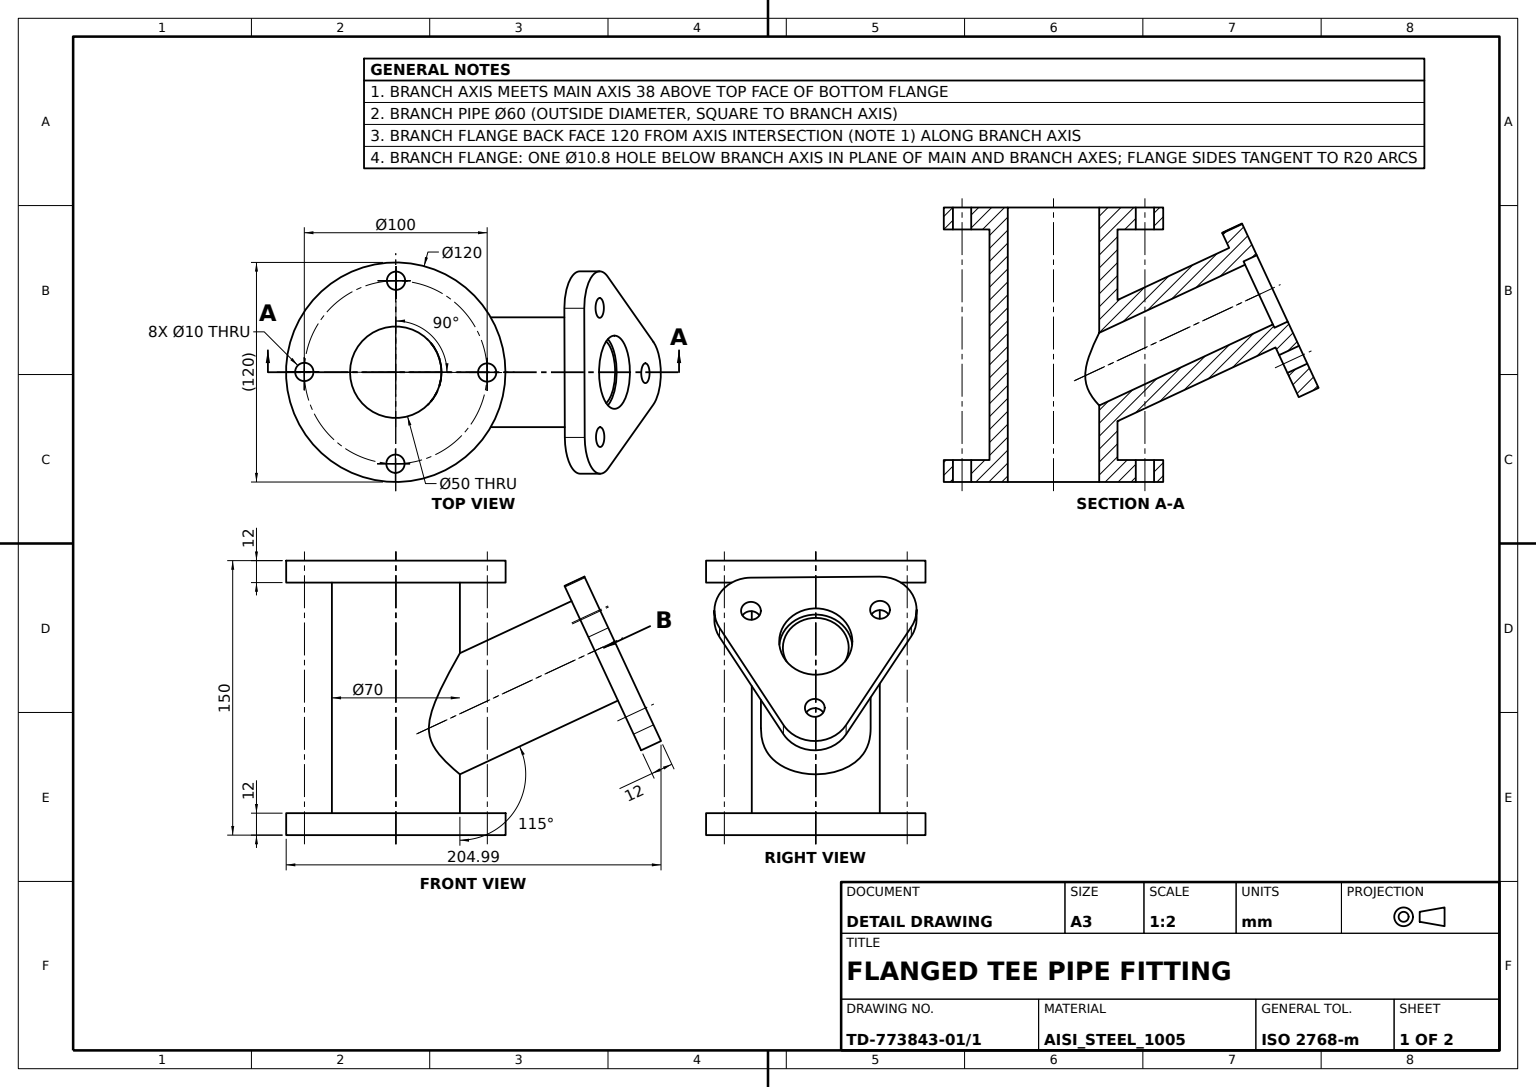
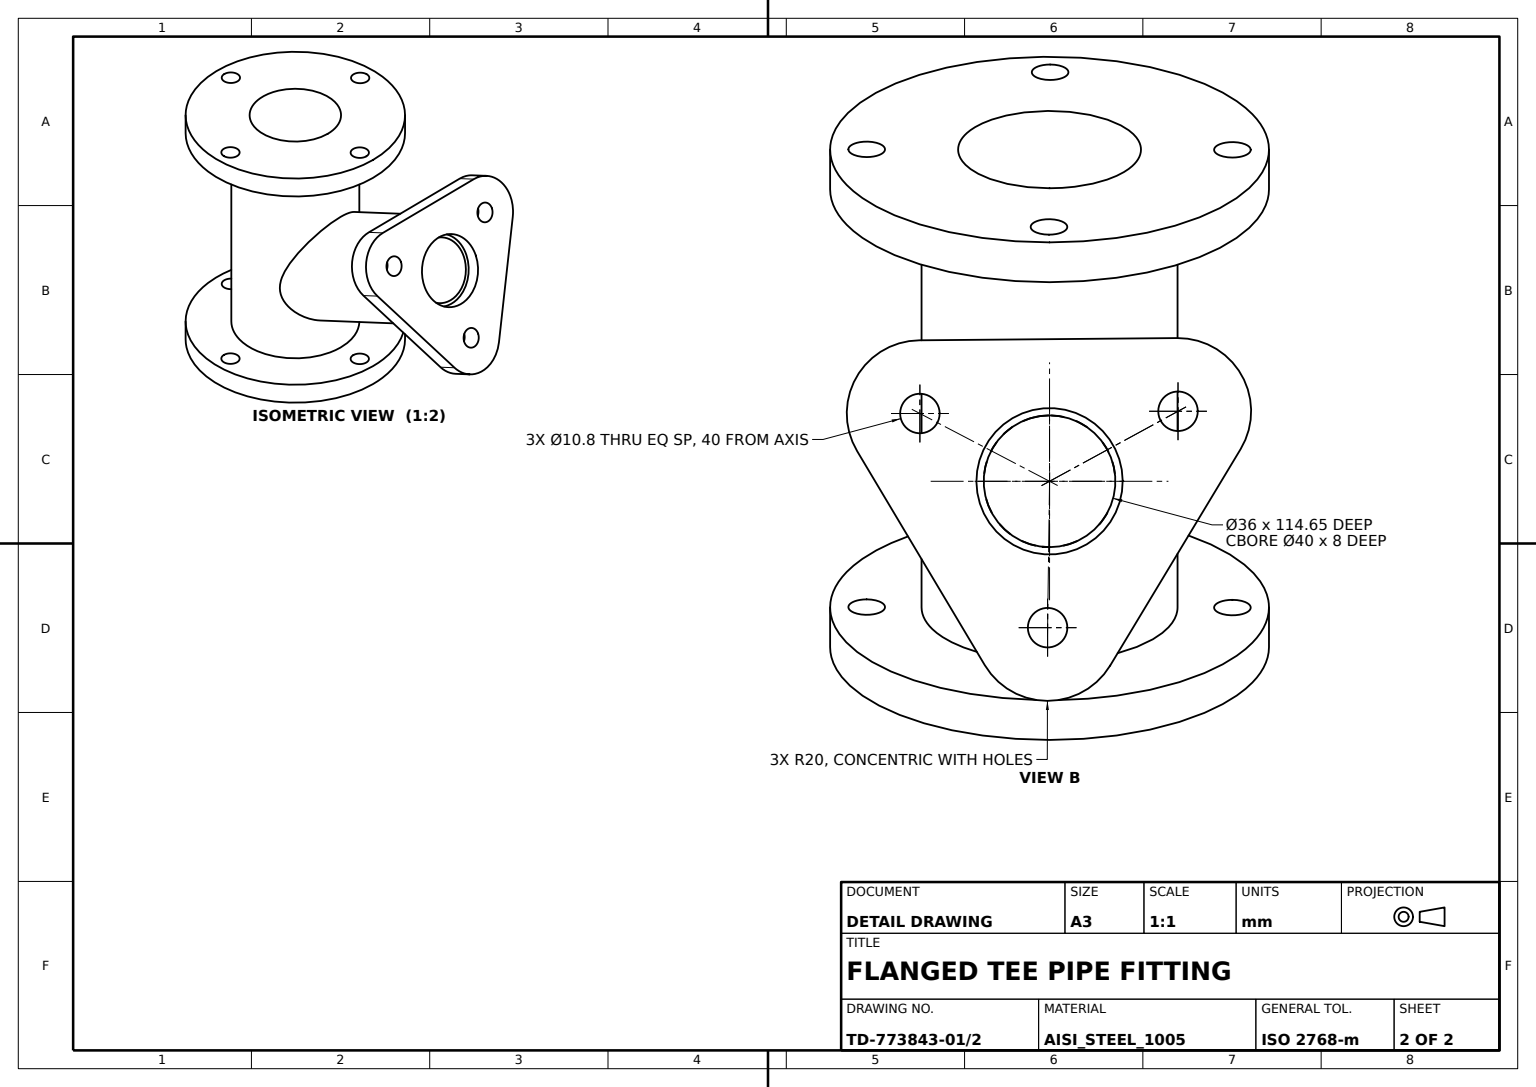
ISO-10303-21;
HEADER;
FILE_DESCRIPTION((''),'2;1');
FILE_NAME('','',(''),(''),'','','');
FILE_SCHEMA(('AUTOMOTIVE_DESIGN'));
ENDSEC;
DATA;
#1=APPLICATION_CONTEXT('');
#2=PRODUCT_CONTEXT('',#1,'mechanical');
#3=PRODUCT('','','',(#2));
#4=PRODUCT_DEFINITION_FORMATION('','',#3);
#5=PRODUCT_DEFINITION_CONTEXT('',#1,'design');
#6=PRODUCT_DEFINITION('','',#4,#5);
#7=PRODUCT_DEFINITION_SHAPE('','',#6);
#8=(LENGTH_UNIT()NAMED_UNIT(*)SI_UNIT(.MILLI.,.METRE.));
#9=(NAMED_UNIT(*)PLANE_ANGLE_UNIT()SI_UNIT($,.RADIAN.));
#10=(NAMED_UNIT(*)SI_UNIT($,.STERADIAN.)SOLID_ANGLE_UNIT());
#11=UNCERTAINTY_MEASURE_WITH_UNIT(LENGTH_MEASURE(0.005),#8,'distance_accuracy_value','');
#12=(GEOMETRIC_REPRESENTATION_CONTEXT(3)GLOBAL_UNCERTAINTY_ASSIGNED_CONTEXT((#11))GLOBAL_UNIT_ASSIGNED_CONTEXT((#8,#9,#10))REPRESENTATION_CONTEXT('',''));
#13=CARTESIAN_POINT('',(140.900901,16.593812,60.175653));
#14=VERTEX_POINT('',#13);
#15=CARTESIAN_POINT('',(130.025207,16.593812,55.104234));
#16=VERTEX_POINT('',#15);
#17=DIRECTION('',(-0.906307787,0.,-0.422618262));
#18=VECTOR('',#17,1000.);
#19=LINE('',#13,#18);
#20=EDGE_CURVE('',#14,#16,#19,.T.);
#21=ORIENTED_EDGE('',*,*,#20,.F.);
#22=CARTESIAN_POINT('',(140.867169,-17.707283,60.247989));
#23=VERTEX_POINT('',#22);
#24=CARTESIAN_POINT('',(136.535859,-0.532795,69.536515));
#25=DIRECTION('',(-0.422618262,0.,0.906307787));
#26=AXIS2_PLACEMENT_3D('',#24,#17,#25);
#27=CIRCLE('',#26,20.);
#28=EDGE_CURVE('',#14,#23,#27,.T.);
#29=ORIENTED_EDGE('',*,*,#28,.T.);
#30=CARTESIAN_POINT('',(129.991476,-17.707283,55.17657));
#31=VERTEX_POINT('',#30);
#32=LINE('',#22,#18);
#33=EDGE_CURVE('',#23,#31,#32,.T.);
#34=ORIENTED_EDGE('',*,*,#33,.T.);
#35=CARTESIAN_POINT('',(125.660165,-0.532795,64.465096));
#36=AXIS2_PLACEMENT_3D('',#35,#17,#25);
#37=CIRCLE('',#36,20.);
#38=EDGE_CURVE('',#16,#31,#37,.T.);
#39=ORIENTED_EDGE('',*,*,#38,.F.);
#40=EDGE_LOOP('',(#21,#29,#34,#39));
#41=FACE_BOUND('',#40,.T.);
#42=CYLINDRICAL_SURFACE('',#26,20.);
#43=ADVANCED_FACE('',(#41),#42,.T.);
#44=CARTESIAN_POINT('',(60.,0.,150.));
#45=VERTEX_POINT('',#44);
#46=CARTESIAN_POINT('',(0.,0.,150.));
#47=DIRECTION('',(0.,0.,1.));
#48=DIRECTION('',(1.,0.,0.));
#49=AXIS2_PLACEMENT_3D('',#46,#47,#48);
#50=CIRCLE('',#49,60.);
#51=EDGE_CURVE('',#45,#45,#50,.T.);
#52=ORIENTED_EDGE('',*,*,#51,.F.);
#53=EDGE_LOOP('',(#52));
#54=FACE_BOUND('',#53,.T.);
#55=CARTESIAN_POINT('',(60.,0.,138.));
#56=VERTEX_POINT('',#55);
#57=CARTESIAN_POINT('',(0.,0.,138.));
#58=AXIS2_PLACEMENT_3D('',#57,#47,#48);
#59=CIRCLE('',#58,60.);
#60=EDGE_CURVE('',#56,#56,#59,.T.);
#61=ORIENTED_EDGE('',*,*,#60,.T.);
#62=EDGE_LOOP('',(#61));
#63=FACE_BOUND('',#62,.T.);
#64=DIRECTION('',(0.,0.,-1.));
#65=DIRECTION('',(-1.,0.,0.));
#66=AXIS2_PLACEMENT_3D('',#46,#64,#65);
#67=CYLINDRICAL_SURFACE('',#66,60.);
#68=ADVANCED_FACE('',(#54,#63),#67,.T.);
#69=CARTESIAN_POINT('',(116.136196,-52.627765,113.283733));
#70=VERTEX_POINT('',#69);
#71=DIRECTION('',(-0.362912611,-0.512437715,0.778268607));
#72=VECTOR('',#71,1000.);
#73=LINE('',#22,#72);
#74=EDGE_CURVE('',#23,#70,#73,.T.);
#75=ORIENTED_EDGE('',*,*,#74,.T.);
#76=CARTESIAN_POINT('',(105.260502,-52.627765,108.212314));
#77=VERTEX_POINT('',#76);
#78=LINE('',#69,#18);
#79=EDGE_CURVE('',#70,#77,#78,.T.);
#80=ORIENTED_EDGE('',*,*,#79,.T.);
#81=LINE('',#30,#72);
#82=EDGE_CURVE('',#31,#77,#81,.T.);
#83=ORIENTED_EDGE('',*,*,#82,.F.);
#84=ORIENTED_EDGE('',*,*,#33,.F.);
#85=EDGE_LOOP('',(#75,#80,#83,#84));
#86=FACE_BOUND('',#85,.T.);
#87=DIRECTION('',(0.216565536,-0.858724396,-0.464426292));
#88=DIRECTION('',(0.,0.475715943,-0.879598966));
#89=AXIS2_PLACEMENT_3D('',#22,#87,#88);
#90=PLANE('',#89);
#91=ADVANCED_FACE('',(#86),#90,.T.);
#92=CARTESIAN_POINT('',(98.388538,35.126926,122.94929));
#93=VERTEX_POINT('',#92);
#94=CARTESIAN_POINT('',(100.670676,35.126926,118.055228));
#95=AXIS2_PLACEMENT_3D('',#94,#17,#25);
#96=CIRCLE('',#95,5.4);
#97=EDGE_CURVE('',#93,#93,#96,.F.);
#98=ORIENTED_EDGE('',*,*,#97,.T.);
#99=EDGE_LOOP('',(#98));
#100=FACE_BOUND('',#99,.T.);
#101=CARTESIAN_POINT('',(123.378027,-0.532795,69.359158));
#102=VERTEX_POINT('',#101);
#103=CIRCLE('',#36,5.4);
#104=EDGE_CURVE('',#102,#102,#103,.F.);
#105=ORIENTED_EDGE('',*,*,#104,.T.);
#106=EDGE_LOOP('',(#105));
#107=FACE_BOUND('',#106,.T.);
#108=CARTESIAN_POINT('',(92.477144,-35.626605,135.626315));
#109=VERTEX_POINT('',#108);
#110=CARTESIAN_POINT('',(100.929192,-35.453277,117.50084));
#111=AXIS2_PLACEMENT_3D('',#110,#17,#25);
#112=CIRCLE('',#111,20.);
#113=EDGE_CURVE('',#77,#109,#112,.T.);
#114=ORIENTED_EDGE('',*,*,#113,.T.);
#115=CARTESIAN_POINT('',(92.218629,34.953598,136.180703));
#116=VERTEX_POINT('',#115);
#117=DIRECTION('',(-0.003662578,0.999962446,0.007854424));
#118=VECTOR('',#117,1000.);
#119=LINE('',#108,#118);
#120=EDGE_CURVE('',#109,#116,#119,.T.);
#121=ORIENTED_EDGE('',*,*,#120,.T.);
#122=CARTESIAN_POINT('',(105.035718,52.253532,108.694365));
#123=VERTEX_POINT('',#122);
#124=CIRCLE('',#95,20.);
#125=EDGE_CURVE('',#116,#123,#124,.T.);
#126=ORIENTED_EDGE('',*,*,#125,.T.);
#127=DIRECTION('',(0.361900843,-0.516428444,-0.776098861));
#128=VECTOR('',#127,1000.);
#129=LINE('',#122,#128);
#130=EDGE_CURVE('',#123,#16,#129,.T.);
#131=ORIENTED_EDGE('',*,*,#130,.T.);
#132=ORIENTED_EDGE('',*,*,#38,.T.);
#133=ORIENTED_EDGE('',*,*,#82,.T.);
#134=EDGE_LOOP('',(#114,#121,#126,#131,#132,#133));
#135=FACE_BOUND('',#134,.T.);
#136=CARTESIAN_POINT('',(96.078387,0.,127.903425));
#137=VERTEX_POINT('',#136);
#138=CARTESIAN_POINT('',(108.756934,0.,100.714191));
#139=AXIS2_PLACEMENT_3D('',#138,#17,#25);
#140=CIRCLE('',#139,30.);
#141=EDGE_CURVE('',#137,#137,#140,.T.);
#142=ORIENTED_EDGE('',*,*,#141,.F.);
#143=EDGE_LOOP('',(#142));
#144=FACE_BOUND('',#143,.T.);
#145=CARTESIAN_POINT('',(98.647053,-35.453277,122.394902));
#146=VERTEX_POINT('',#145);
#147=CIRCLE('',#111,5.4);
#148=EDGE_CURVE('',#146,#146,#147,.F.);
#149=ORIENTED_EDGE('',*,*,#148,.T.);
#150=EDGE_LOOP('',(#149));
#151=FACE_BOUND('',#150,.T.);
#152=PLANE('',#36);
#153=ADVANCED_FACE('',(#100,#107,#135,#144,#151),#152,.T.);
#154=CARTESIAN_POINT('',(35.,0.,99.422106));
#155=VERTEX_POINT('',#154);
#156=CARTESIAN_POINT('',(34.892666,3.336117,99.233995));
#157=CARTESIAN_POINT('',(35.053937,0.002477,99.516636));
#158=CARTESIAN_POINT('',(34.891586,-3.346026,99.232095));
#159=CARTESIAN_POINT('',(34.432516,-6.541423,98.42562));
#160=CARTESIAN_POINT('',(33.706124,-9.588786,97.143219));
#161=CARTESIAN_POINT('',(32.790064,-12.348332,95.514214));
#162=CARTESIAN_POINT('',(31.710242,-14.893669,93.575005));
#163=CARTESIAN_POINT('',(30.539362,-17.156852,91.445453));
#164=CARTESIAN_POINT('',(29.292957,-19.202714,89.142785));
#165=CARTESIAN_POINT('',(27.54659,-21.679761,85.851269));
#166=CARTESIAN_POINT('',(25.313683,-24.271143,81.483274));
#167=CARTESIAN_POINT('',(22.694251,-26.714562,75.932155));
#168=CARTESIAN_POINT('',(20.26603,-28.579234,69.980266));
#169=CARTESIAN_POINT('',(18.369665,-29.803927,63.661125));
#170=CARTESIAN_POINT('',(17.813466,-30.127869,58.07606));
#171=CARTESIAN_POINT('',(18.489088,-29.722367,53.660067));
#172=CARTESIAN_POINT('',(19.912625,-28.814185,49.502577));
#173=CARTESIAN_POINT('',(22.737038,-26.751124,45.04564));
#174=CARTESIAN_POINT('',(25.830517,-23.745952,41.573159));
#175=CARTESIAN_POINT('',(28.211912,-20.782049,39.194022));
#176=CARTESIAN_POINT('',(29.854607,-18.348469,37.653808));
#177=CARTESIAN_POINT('',(31.341958,-15.68269,36.319432));
#178=CARTESIAN_POINT('',(33.06183,-11.820999,34.828032));
#179=CARTESIAN_POINT('',(34.263533,-7.717586,33.826214));
#180=CARTESIAN_POINT('',(34.89825,-3.2939,33.302789));
#181=CARTESIAN_POINT('',(35.051649,0.012345,33.177116));
#182=CARTESIAN_POINT('',(34.895139,3.326243,33.305345));
#183=CARTESIAN_POINT('',(34.258225,7.74275,33.830606));
#184=CARTESIAN_POINT('',(33.040853,11.883005,34.845614));
#185=CARTESIAN_POINT('',(31.312657,15.739341,36.345367));
#186=CARTESIAN_POINT('',(29.336743,19.272218,38.118779));
#187=CARTESIAN_POINT('',(26.416762,23.182953,40.911858));
#188=CARTESIAN_POINT('',(22.699576,26.782139,45.09296));
#189=CARTESIAN_POINT('',(19.884807,28.83293,49.55745));
#190=CARTESIAN_POINT('',(18.477352,29.729316,53.713564));
#191=CARTESIAN_POINT('',(17.981047,30.028031,56.999503));
#192=CARTESIAN_POINT('',(18.038018,29.994213,60.3695));
#193=CARTESIAN_POINT('',(18.530554,29.695439,63.648904));
#194=CARTESIAN_POINT('',(19.337281,29.179937,66.873262));
#195=CARTESIAN_POINT('',(20.674578,28.264222,70.984292));
#196=CARTESIAN_POINT('',(22.689441,26.720083,75.921614));
#197=CARTESIAN_POINT('',(25.339611,24.244773,81.536819));
#198=CARTESIAN_POINT('',(28.002114,21.148324,86.740889));
#199=CARTESIAN_POINT('',(30.163285,17.888984,90.761934));
#200=CARTESIAN_POINT('',(31.722995,14.86602,93.597992));
#201=CARTESIAN_POINT('',(32.798427,12.32605,95.529139));
#202=CARTESIAN_POINT('',(33.710295,9.57138,97.150583));
#203=CARTESIAN_POINT('',(34.430491,6.55201,98.422049));
#204=B_SPLINE_CURVE_WITH_KNOTS('',3,(#156,#157,#158,#159,#160,#161,#162,#163,#164,#165,#166,#167,#168,#169,#170,#171,#172,#173,#174,#175,#176,#177,#178,#179,#180,#181,#182,#183,#184,#185,#186,#187,#188,#189,#190,#191,#192,#193,#194,#195,#196,#197,#198,#199,#200,#201,#202,#203,#156,#157,#158),.UNSPECIFIED.,.T.,.F.,(1,1,1,1,1,1,1,1,1,1,1,1,1,1,1,1,1,1,1,1,1,1,1,1,1,1,1,1,1,1,1,1,1,1,1,1,1,1,1,1,1,1,1,1,1,1,1,1,1,1,1,1,1,1,1),(-0.009948517,-0.006632345,-0.003316172,0.,0.003316172,0.006632345,0.009948517,0.01326469,0.016580862,0.019897034,0.023213207,0.026529379,0.033161724,0.039794069,0.046426414,0.053058758,0.059691103,0.063007276,0.066323448,0.072955793,0.079588137,0.08290431,0.086220482,0.089536655,0.092852827,0.099485172,0.102801344,0.106117517,0.109433689,0.112749861,0.119382206,0.122698379,0.126014551,0.132646896,0.139279241,0.145911585,0.149227758,0.15254393,0.155860103,0.159176275,0.162492447,0.16580862,0.172440965,0.179073309,0.185705654,0.192337999,0.195654171,0.198970344,0.202286516,0.205602689,0.208918861,0.212235033,0.215551206,0.218867378,0.222183551),.UNSPECIFIED.);
#205=EDGE_CURVE('',#155,#155,#204,.T.);
#206=ORIENTED_EDGE('',*,*,#205,.T.);
#207=EDGE_LOOP('',(#206));
#208=FACE_BOUND('',#207,.T.);
#209=ORIENTED_EDGE('',*,*,#141,.T.);
#210=EDGE_LOOP('',(#209));
#211=FACE_BOUND('',#210,.T.);
#212=CYLINDRICAL_SURFACE('',#139,30.);
#213=ADVANCED_FACE('',(#208,#211),#212,.T.);
#214=CARTESIAN_POINT('',(-0.154889,-54.99976,150.));
#215=VERTEX_POINT('',#214);
#216=CARTESIAN_POINT('',(-0.154889,-49.99976,150.));
#217=DIRECTION('',(0.,-1.,0.));
#218=AXIS2_PLACEMENT_3D('',#216,#64,#217);
#219=CIRCLE('',#218,5.);
#220=EDGE_CURVE('',#215,#215,#219,.T.);
#221=ORIENTED_EDGE('',*,*,#220,.T.);
#222=EDGE_LOOP('',(#221));
#223=FACE_BOUND('',#222,.T.);
#224=ORIENTED_EDGE('',*,*,#51,.T.);
#225=EDGE_LOOP('',(#224));
#226=FACE_BOUND('',#225,.T.);
#227=CARTESIAN_POINT('',(0.154889,54.99976,150.));
#228=VERTEX_POINT('',#227);
#229=CARTESIAN_POINT('',(0.154889,49.99976,150.));
#230=DIRECTION('',(0.,1.,0.));
#231=AXIS2_PLACEMENT_3D('',#229,#64,#230);
#232=CIRCLE('',#231,5.);
#233=EDGE_CURVE('',#228,#228,#232,.T.);
#234=ORIENTED_EDGE('',*,*,#233,.T.);
#235=EDGE_LOOP('',(#234));
#236=FACE_BOUND('',#235,.T.);
#237=CARTESIAN_POINT('',(-54.99976,0.154889,150.));
#238=VERTEX_POINT('',#237);
#239=CARTESIAN_POINT('',(-49.99976,0.154889,150.));
#240=AXIS2_PLACEMENT_3D('',#239,#64,#65);
#241=CIRCLE('',#240,5.);
#242=EDGE_CURVE('',#238,#238,#241,.T.);
#243=ORIENTED_EDGE('',*,*,#242,.T.);
#244=EDGE_LOOP('',(#243));
#245=FACE_BOUND('',#244,.T.);
#246=CARTESIAN_POINT('',(54.99976,-0.154889,150.));
#247=VERTEX_POINT('',#246);
#248=CARTESIAN_POINT('',(49.99976,-0.154889,150.));
#249=AXIS2_PLACEMENT_3D('',#248,#64,#48);
#250=CIRCLE('',#249,5.);
#251=EDGE_CURVE('',#247,#247,#250,.T.);
#252=ORIENTED_EDGE('',*,*,#251,.T.);
#253=EDGE_LOOP('',(#252));
#254=FACE_BOUND('',#253,.T.);
#255=CARTESIAN_POINT('',(25.,0.,150.));
#256=VERTEX_POINT('',#255);
#257=AXIS2_PLACEMENT_3D('',#46,#64,#48);
#258=CIRCLE('',#257,25.);
#259=EDGE_CURVE('',#256,#256,#258,.T.);
#260=ORIENTED_EDGE('',*,*,#259,.T.);
#261=EDGE_LOOP('',(#260));
#262=FACE_BOUND('',#261,.T.);
#263=PLANE('',#49);
#264=ADVANCED_FACE('',(#223,#226,#236,#245,#254,#262),#263,.T.);
#265=CARTESIAN_POINT('',(-0.154889,-54.99976,0.));
#266=VERTEX_POINT('',#265);
#267=CARTESIAN_POINT('',(-0.154889,-49.99976,0.));
#268=AXIS2_PLACEMENT_3D('',#267,#64,#217);
#269=CIRCLE('',#268,5.);
#270=EDGE_CURVE('',#266,#266,#269,.T.);
#271=ORIENTED_EDGE('',*,*,#270,.T.);
#272=EDGE_LOOP('',(#271));
#273=FACE_BOUND('',#272,.T.);
#274=CARTESIAN_POINT('',(-5.154889,-49.99976,12.));
#275=VERTEX_POINT('',#274);
#276=CARTESIAN_POINT('',(-0.154889,-49.99976,12.));
#277=AXIS2_PLACEMENT_3D('',#276,#64,#65);
#278=CIRCLE('',#277,5.);
#279=EDGE_CURVE('',#275,#275,#278,.F.);
#280=ORIENTED_EDGE('',*,*,#279,.T.);
#281=EDGE_LOOP('',(#280));
#282=FACE_BOUND('',#281,.T.);
#283=AXIS2_PLACEMENT_3D('',#267,#47,#48);
#284=CYLINDRICAL_SURFACE('',#283,5.);
#285=ADVANCED_FACE('',(#273,#282),#284,.F.);
#286=CARTESIAN_POINT('',(103.094322,34.953598,141.252122));
#287=VERTEX_POINT('',#286);
#288=CARTESIAN_POINT('',(115.911412,52.253532,113.765784));
#289=VERTEX_POINT('',#288);
#290=CARTESIAN_POINT('',(111.54637,35.126926,123.126647));
#291=AXIS2_PLACEMENT_3D('',#290,#17,#25);
#292=CIRCLE('',#291,20.);
#293=EDGE_CURVE('',#287,#289,#292,.T.);
#294=ORIENTED_EDGE('',*,*,#293,.T.);
#295=LINE('',#288,#18);
#296=EDGE_CURVE('',#289,#123,#295,.T.);
#297=ORIENTED_EDGE('',*,*,#296,.T.);
#298=ORIENTED_EDGE('',*,*,#125,.F.);
#299=LINE('',#286,#18);
#300=EDGE_CURVE('',#287,#116,#299,.T.);
#301=ORIENTED_EDGE('',*,*,#300,.F.);
#302=EDGE_LOOP('',(#294,#297,#298,#301));
#303=FACE_BOUND('',#302,.T.);
#304=CYLINDRICAL_SURFACE('',#291,20.);
#305=ADVANCED_FACE('',(#303),#304,.T.);
#306=CARTESIAN_POINT('',(35.,0.,12.));
#307=VERTEX_POINT('',#306);
#308=CARTESIAN_POINT('',(0.,0.,12.));
#309=AXIS2_PLACEMENT_3D('',#308,#47,#48);
#310=CIRCLE('',#309,35.);
#311=EDGE_CURVE('',#307,#307,#310,.T.);
#312=ORIENTED_EDGE('',*,*,#311,.T.);
#313=EDGE_LOOP('',(#312));
#314=FACE_BOUND('',#313,.T.);
#315=CARTESIAN_POINT('',(35.,0.,138.));
#316=VERTEX_POINT('',#315);
#317=CIRCLE('',#58,35.);
#318=EDGE_CURVE('',#316,#316,#317,.T.);
#319=ORIENTED_EDGE('',*,*,#318,.F.);
#320=EDGE_LOOP('',(#319));
#321=FACE_BOUND('',#320,.T.);
#322=ORIENTED_EDGE('',*,*,#205,.F.);
#323=EDGE_LOOP('',(#322));
#324=FACE_BOUND('',#323,.T.);
#325=AXIS2_PLACEMENT_3D('',#57,#64,#65);
#326=CYLINDRICAL_SURFACE('',#325,35.);
#327=ADVANCED_FACE('',(#314,#321,#324),#326,.T.);
#328=CARTESIAN_POINT('',(111.526592,40.526723,123.169061));
#329=VERTEX_POINT('',#328);
#330=AXIS2_PLACEMENT_3D('',#290,#17,#117);
#331=CIRCLE('',#330,5.4);
#332=EDGE_CURVE('',#329,#329,#331,.T.);
#333=ORIENTED_EDGE('',*,*,#332,.F.);
#334=EDGE_LOOP('',(#333));
#335=FACE_BOUND('',#334,.T.);
#336=ORIENTED_EDGE('',*,*,#97,.F.);
#337=EDGE_LOOP('',(#336));
#338=FACE_BOUND('',#337,.T.);
#339=CARTESIAN_POINT('',(93.420214,35.126926,114.674281));
#340=DIRECTION('',(0.906307787,0.,0.422618262));
#341=DIRECTION('',(0.422618262,0.,-0.906307787));
#342=AXIS2_PLACEMENT_3D('',#339,#340,#341);
#343=CYLINDRICAL_SURFACE('',#342,5.4);
#344=ADVANCED_FACE('',(#335,#338),#343,.F.);
#345=CARTESIAN_POINT('',(-44.99976,0.154889,138.));
#346=VERTEX_POINT('',#345);
#347=CARTESIAN_POINT('',(-49.99976,0.154889,138.));
#348=AXIS2_PLACEMENT_3D('',#347,#47,#48);
#349=CIRCLE('',#348,5.);
#350=EDGE_CURVE('',#346,#346,#349,.F.);
#351=ORIENTED_EDGE('',*,*,#350,.T.);
#352=EDGE_LOOP('',(#351));
#353=FACE_BOUND('',#352,.T.);
#354=ORIENTED_EDGE('',*,*,#242,.F.);
#355=EDGE_LOOP('',(#354));
#356=FACE_BOUND('',#355,.T.);
#357=CARTESIAN_POINT('',(-49.99976,0.154889,0.));
#358=AXIS2_PLACEMENT_3D('',#357,#47,#48);
#359=CYLINDRICAL_SURFACE('',#358,5.);
#360=ADVANCED_FACE('',(#353,#356),#359,.F.);
#361=CARTESIAN_POINT('',(25.,0.,41.796889));
#362=VERTEX_POINT('',#361);
#363=CARTESIAN_POINT('',(24.948579,-1.952403,41.851562));
#364=CARTESIAN_POINT('',(25.050927,0.655099,41.742861));
#365=CARTESIAN_POINT('',(24.79876,3.866121,42.009774));
#366=CARTESIAN_POINT('',(23.922568,7.569045,42.967034));
#367=CARTESIAN_POINT('',(22.59564,10.877432,44.525663));
#368=CARTESIAN_POINT('',(20.986023,13.700118,46.668299));
#369=CARTESIAN_POINT('',(19.594578,15.560459,48.977225));
#370=CARTESIAN_POINT('',(18.639925,16.669856,51.097068));
#371=CARTESIAN_POINT('',(17.834655,17.532507,53.438358));
#372=CARTESIAN_POINT('',(17.385279,17.965047,55.946107));
#373=CARTESIAN_POINT('',(17.32576,18.022778,58.56502));
#374=CARTESIAN_POINT('',(17.495911,17.858815,61.123786));
#375=CARTESIAN_POINT('',(18.072814,17.288475,64.296085));
#376=CARTESIAN_POINT('',(19.09347,16.169485,67.829369));
#377=CARTESIAN_POINT('',(20.310346,14.629764,71.19497));
#378=CARTESIAN_POINT('',(21.5884,12.688348,74.28318));
#379=CARTESIAN_POINT('',(22.832547,10.317957,77.048713));
#380=CARTESIAN_POINT('',(23.958755,7.3961,79.415619));
#381=CARTESIAN_POINT('',(24.783499,3.935884,81.087443));
#382=CARTESIAN_POINT('',(25.104143,0.048307,81.72577));
#383=CARTESIAN_POINT('',(24.799649,-3.838276,81.119877));
#384=CARTESIAN_POINT('',(23.980441,-7.324801,79.459838));
#385=CARTESIAN_POINT('',(22.872667,-10.230021,77.135299));
#386=CARTESIAN_POINT('',(21.611783,-12.650767,74.337389));
#387=CARTESIAN_POINT('',(20.339012,-14.589672,71.26799));
#388=CARTESIAN_POINT('',(19.113622,-16.146262,67.891544));
#389=CARTESIAN_POINT('',(18.091778,-17.268908,64.369456));
#390=CARTESIAN_POINT('',(17.389964,-17.963236,60.582117));
#391=CARTESIAN_POINT('',(17.286261,-18.061136,57.33033));
#392=CARTESIAN_POINT('',(17.599197,-17.757748,54.745834));
#393=CARTESIAN_POINT('',(18.159575,-17.193047,52.300072));
#394=CARTESIAN_POINT('',(19.298634,-15.953767,49.465026));
#395=CARTESIAN_POINT('',(20.967503,-13.729445,46.696648));
#396=CARTESIAN_POINT('',(22.592458,-10.885075,44.528477));
#397=CARTESIAN_POINT('',(23.918556,-7.582738,42.971905));
#398=CARTESIAN_POINT('',(24.652859,-4.481901,42.168933));
#399=B_SPLINE_CURVE_WITH_KNOTS('',3,(#363,#364,#365,#366,#367,#368,#369,#370,#371,#372,#373,#374,#375,#376,#377,#378,#379,#380,#381,#382,#383,#384,#385,#386,#387,#388,#389,#390,#391,#392,#393,#394,#395,#396,#397,#398,#363,#364,#365),.UNSPECIFIED.,.T.,.F.,(1,1,1,1,1,1,1,1,1,1,1,1,1,1,1,1,1,1,1,1,1,1,1,1,1,1,1,1,1,1,1,1,1,1,1,1,1,1,1,1,1,1,1),(-0.007717956,-0.003858978,-0.001929489,0.,0.003858978,0.007717956,0.011576935,0.015435913,0.019294891,0.02122438,0.023153869,0.027012847,0.028942337,0.030871826,0.034730804,0.038589782,0.04244876,0.046307739,0.050166717,0.054025695,0.057884673,0.061743651,0.06560263,0.069461608,0.073320586,0.077179564,0.081038542,0.084897521,0.088756499,0.092615477,0.096474455,0.098403944,0.100333434,0.104192412,0.10805139,0.111910368,0.115769346,0.119628325,0.121557814,0.123487303,0.127346281,0.131205259,0.135064237),.UNSPECIFIED.);
#400=EDGE_CURVE('',#362,#362,#399,.T.);
#401=ORIENTED_EDGE('',*,*,#400,.F.);
#402=EDGE_LOOP('',(#401));
#403=FACE_BOUND('',#402,.T.);
#404=CARTESIAN_POINT('',(104.775037,0.,118.718205));
#405=VERTEX_POINT('',#404);
#406=CARTESIAN_POINT('',(112.382166,0.,102.404664));
#407=AXIS2_PLACEMENT_3D('',#406,#17,#25);
#408=CIRCLE('',#407,18.);
#409=EDGE_CURVE('',#405,#405,#408,.F.);
#410=ORIENTED_EDGE('',*,*,#409,.T.);
#411=EDGE_LOOP('',(#410));
#412=FACE_BOUND('',#411,.T.);
#413=CARTESIAN_POINT('',(10.875693,0.,55.071419));
#414=AXIS2_PLACEMENT_3D('',#413,#340,#341);
#415=CYLINDRICAL_SURFACE('',#414,18.);
#416=ADVANCED_FACE('',(#403,#412),#415,.F.);
#417=CARTESIAN_POINT('',(44.99976,-0.154889,12.));
#418=VERTEX_POINT('',#417);
#419=CARTESIAN_POINT('',(49.99976,-0.154889,12.));
#420=AXIS2_PLACEMENT_3D('',#419,#64,#65);
#421=CIRCLE('',#420,5.);
#422=EDGE_CURVE('',#418,#418,#421,.F.);
#423=ORIENTED_EDGE('',*,*,#422,.T.);
#424=EDGE_LOOP('',(#423));
#425=FACE_BOUND('',#424,.T.);
#426=CARTESIAN_POINT('',(54.99976,-0.154889,0.));
#427=VERTEX_POINT('',#426);
#428=CARTESIAN_POINT('',(49.99976,-0.154889,0.));
#429=AXIS2_PLACEMENT_3D('',#428,#64,#48);
#430=CIRCLE('',#429,5.);
#431=EDGE_CURVE('',#427,#427,#430,.T.);
#432=ORIENTED_EDGE('',*,*,#431,.T.);
#433=EDGE_LOOP('',(#432));
#434=FACE_BOUND('',#433,.T.);
#435=AXIS2_PLACEMENT_3D('',#428,#47,#48);
#436=CYLINDRICAL_SURFACE('',#435,5.);
#437=ADVANCED_FACE('',(#425,#434),#436,.F.);
#438=CARTESIAN_POINT('',(60.,0.,12.));
#439=VERTEX_POINT('',#438);
#440=AXIS2_PLACEMENT_3D('',#308,#64,#48);
#441=CIRCLE('',#440,60.);
#442=EDGE_CURVE('',#439,#439,#441,.T.);
#443=ORIENTED_EDGE('',*,*,#442,.T.);
#444=EDGE_LOOP('',(#443));
#445=FACE_BOUND('',#444,.T.);
#446=CARTESIAN_POINT('',(60.,0.,0.));
#447=VERTEX_POINT('',#446);
#448=CARTESIAN_POINT('',(0.,0.,0.));
#449=AXIS2_PLACEMENT_3D('',#448,#64,#48);
#450=CIRCLE('',#449,60.);
#451=EDGE_CURVE('',#447,#447,#450,.T.);
#452=ORIENTED_EDGE('',*,*,#451,.F.);
#453=EDGE_LOOP('',(#452));
#454=FACE_BOUND('',#453,.T.);
#455=AXIS2_PLACEMENT_3D('',#308,#64,#65);
#456=CYLINDRICAL_SURFACE('',#455,60.);
#457=ADVANCED_FACE('',(#445,#454),#456,.T.);
#458=CARTESIAN_POINT('',(-54.99976,0.154889,12.));
#459=VERTEX_POINT('',#458);
#460=CARTESIAN_POINT('',(-49.99976,0.154889,12.));
#461=AXIS2_PLACEMENT_3D('',#460,#64,#65);
#462=CIRCLE('',#461,5.);
#463=EDGE_CURVE('',#459,#459,#462,.F.);
#464=ORIENTED_EDGE('',*,*,#463,.T.);
#465=EDGE_LOOP('',(#464));
#466=FACE_BOUND('',#465,.T.);
#467=CARTESIAN_POINT('',(-54.99976,0.154889,0.));
#468=VERTEX_POINT('',#467);
#469=AXIS2_PLACEMENT_3D('',#357,#64,#65);
#470=CIRCLE('',#469,5.);
#471=EDGE_CURVE('',#468,#468,#470,.T.);
#472=ORIENTED_EDGE('',*,*,#471,.T.);
#473=EDGE_LOOP('',(#472));
#474=FACE_BOUND('',#473,.T.);
#475=ADVANCED_FACE('',(#466,#474),#359,.F.);
#476=ORIENTED_EDGE('',*,*,#318,.T.);
#477=EDGE_LOOP('',(#476));
#478=FACE_BOUND('',#477,.T.);
#479=CARTESIAN_POINT('',(54.99976,-0.154889,138.));
#480=VERTEX_POINT('',#479);
#481=CARTESIAN_POINT('',(49.99976,-0.154889,138.));
#482=AXIS2_PLACEMENT_3D('',#481,#47,#48);
#483=CIRCLE('',#482,5.);
#484=EDGE_CURVE('',#480,#480,#483,.F.);
#485=ORIENTED_EDGE('',*,*,#484,.F.);
#486=EDGE_LOOP('',(#485));
#487=FACE_BOUND('',#486,.T.);
#488=ORIENTED_EDGE('',*,*,#350,.F.);
#489=EDGE_LOOP('',(#488));
#490=FACE_BOUND('',#489,.T.);
#491=ORIENTED_EDGE('',*,*,#60,.F.);
#492=EDGE_LOOP('',(#491));
#493=FACE_BOUND('',#492,.T.);
#494=CARTESIAN_POINT('',(5.154889,49.99976,138.));
#495=VERTEX_POINT('',#494);
#496=CARTESIAN_POINT('',(0.154889,49.99976,138.));
#497=AXIS2_PLACEMENT_3D('',#496,#47,#48);
#498=CIRCLE('',#497,5.);
#499=EDGE_CURVE('',#495,#495,#498,.F.);
#500=ORIENTED_EDGE('',*,*,#499,.F.);
#501=EDGE_LOOP('',(#500));
#502=FACE_BOUND('',#501,.T.);
#503=CARTESIAN_POINT('',(4.845111,-49.99976,138.));
#504=VERTEX_POINT('',#503);
#505=CARTESIAN_POINT('',(-0.154889,-49.99976,138.));
#506=AXIS2_PLACEMENT_3D('',#505,#47,#48);
#507=CIRCLE('',#506,5.);
#508=EDGE_CURVE('',#504,#504,#507,.F.);
#509=ORIENTED_EDGE('',*,*,#508,.F.);
#510=EDGE_LOOP('',(#509));
#511=FACE_BOUND('',#510,.T.);
#512=PLANE('',#58);
#513=ADVANCED_FACE('',(#478,#487,#490,#493,#502,#511),#512,.F.);
#514=ORIENTED_EDGE('',*,*,#442,.F.);
#515=EDGE_LOOP('',(#514));
#516=FACE_BOUND('',#515,.T.);
#517=CARTESIAN_POINT('',(-4.845111,49.99976,12.));
#518=VERTEX_POINT('',#517);
#519=CARTESIAN_POINT('',(0.154889,49.99976,12.));
#520=AXIS2_PLACEMENT_3D('',#519,#64,#65);
#521=CIRCLE('',#520,5.);
#522=EDGE_CURVE('',#518,#518,#521,.F.);
#523=ORIENTED_EDGE('',*,*,#522,.F.);
#524=EDGE_LOOP('',(#523));
#525=FACE_BOUND('',#524,.T.);
#526=ORIENTED_EDGE('',*,*,#463,.F.);
#527=EDGE_LOOP('',(#526));
#528=FACE_BOUND('',#527,.T.);
#529=ORIENTED_EDGE('',*,*,#311,.F.);
#530=EDGE_LOOP('',(#529));
#531=FACE_BOUND('',#530,.T.);
#532=ORIENTED_EDGE('',*,*,#422,.F.);
#533=EDGE_LOOP('',(#532));
#534=FACE_BOUND('',#533,.T.);
#535=ORIENTED_EDGE('',*,*,#279,.F.);
#536=EDGE_LOOP('',(#535));
#537=FACE_BOUND('',#536,.T.);
#538=PLANE('',#455);
#539=ADVANCED_FACE('',(#516,#525,#528,#531,#534,#537),#538,.F.);
#540=ORIENTED_EDGE('',*,*,#431,.F.);
#541=EDGE_LOOP('',(#540));
#542=FACE_BOUND('',#541,.T.);
#543=ORIENTED_EDGE('',*,*,#270,.F.);
#544=EDGE_LOOP('',(#543));
#545=FACE_BOUND('',#544,.T.);
#546=CARTESIAN_POINT('',(0.154889,54.99976,0.));
#547=VERTEX_POINT('',#546);
#548=CARTESIAN_POINT('',(0.154889,49.99976,0.));
#549=AXIS2_PLACEMENT_3D('',#548,#64,#230);
#550=CIRCLE('',#549,5.);
#551=EDGE_CURVE('',#547,#547,#550,.T.);
#552=ORIENTED_EDGE('',*,*,#551,.F.);
#553=EDGE_LOOP('',(#552));
#554=FACE_BOUND('',#553,.T.);
#555=CARTESIAN_POINT('',(25.,0.,0.));
#556=VERTEX_POINT('',#555);
#557=CIRCLE('',#449,25.);
#558=EDGE_CURVE('',#556,#556,#557,.T.);
#559=ORIENTED_EDGE('',*,*,#558,.F.);
#560=EDGE_LOOP('',(#559));
#561=FACE_BOUND('',#560,.T.);
#562=ORIENTED_EDGE('',*,*,#471,.F.);
#563=EDGE_LOOP('',(#562));
#564=FACE_BOUND('',#563,.T.);
#565=ORIENTED_EDGE('',*,*,#451,.T.);
#566=EDGE_LOOP('',(#565));
#567=FACE_BOUND('',#566,.T.);
#568=AXIS2_PLACEMENT_3D('',#448,#64,#65);
#569=PLANE('',#568);
#570=ADVANCED_FACE('',(#542,#545,#554,#561,#564,#567),#569,.T.);
#571=ORIENTED_EDGE('',*,*,#499,.T.);
#572=EDGE_LOOP('',(#571));
#573=FACE_BOUND('',#572,.T.);
#574=ORIENTED_EDGE('',*,*,#233,.F.);
#575=EDGE_LOOP('',(#574));
#576=FACE_BOUND('',#575,.T.);
#577=AXIS2_PLACEMENT_3D('',#548,#47,#48);
#578=CYLINDRICAL_SURFACE('',#577,5.);
#579=ADVANCED_FACE('',(#573,#576),#578,.F.);
#580=ORIENTED_EDGE('',*,*,#296,.F.);
#581=LINE('',#288,#128);
#582=EDGE_CURVE('',#289,#14,#581,.T.);
#583=ORIENTED_EDGE('',*,*,#582,.T.);
#584=ORIENTED_EDGE('',*,*,#20,.T.);
#585=ORIENTED_EDGE('',*,*,#130,.F.);
#586=EDGE_LOOP('',(#580,#583,#584,#585));
#587=FACE_BOUND('',#586,.T.);
#588=DIRECTION('',(0.218252091,0.856330347,-0.46804312));
#589=DIRECTION('',(0.,0.479605239,0.877484367));
#590=AXIS2_PLACEMENT_3D('',#288,#588,#589);
#591=PLANE('',#590);
#592=ADVANCED_FACE('',(#587),#591,.T.);
#593=CARTESIAN_POINT('',(103.352837,-35.626605,140.697734));
#594=VERTEX_POINT('',#593);
#595=LINE('',#593,#18);
#596=EDGE_CURVE('',#594,#109,#595,.T.);
#597=ORIENTED_EDGE('',*,*,#596,.F.);
#598=LINE('',#593,#118);
#599=EDGE_CURVE('',#594,#287,#598,.T.);
#600=ORIENTED_EDGE('',*,*,#599,.T.);
#601=ORIENTED_EDGE('',*,*,#300,.T.);
#602=ORIENTED_EDGE('',*,*,#120,.F.);
#603=EDGE_LOOP('',(#597,#600,#601,#602));
#604=FACE_BOUND('',#603,.T.);
#605=DIRECTION('',(-0.422602391,-0.008666398,0.906273752));
#606=AXIS2_PLACEMENT_3D('',#593,#605,#340);
#607=PLANE('',#606);
#608=ADVANCED_FACE('',(#604),#607,.T.);
#609=CARTESIAN_POINT('',(119.559376,19.999249,105.942699));
#610=VERTEX_POINT('',#609);
#611=CARTESIAN_POINT('',(119.632628,0.,105.785611));
#612=AXIS2_PLACEMENT_3D('',#611,#17,#117);
#613=CIRCLE('',#612,20.);
#614=EDGE_CURVE('',#610,#610,#613,.T.);
#615=ORIENTED_EDGE('',*,*,#614,.F.);
#616=EDGE_LOOP('',(#615));
#617=FACE_BOUND('',#616,.T.);
#618=CARTESIAN_POINT('',(112.308914,19.999249,102.561753));
#619=VERTEX_POINT('',#618);
#620=AXIS2_PLACEMENT_3D('',#406,#17,#117);
#621=CIRCLE('',#620,20.);
#622=EDGE_CURVE('',#619,#619,#621,.F.);
#623=ORIENTED_EDGE('',*,*,#622,.F.);
#624=EDGE_LOOP('',(#623));
#625=FACE_BOUND('',#624,.T.);
#626=AXIS2_PLACEMENT_3D('',#406,#340,#341);
#627=CYLINDRICAL_SURFACE('',#626,20.);
#628=ADVANCED_FACE('',(#617,#625),#627,.F.);
#629=ORIENTED_EDGE('',*,*,#409,.F.);
#630=EDGE_LOOP('',(#629));
#631=FACE_BOUND('',#630,.T.);
#632=ORIENTED_EDGE('',*,*,#622,.T.);
#633=EDGE_LOOP('',(#632));
#634=FACE_BOUND('',#633,.T.);
#635=PLANE('',#407);
#636=ADVANCED_FACE('',(#631,#634),#635,.F.);
#637=ORIENTED_EDGE('',*,*,#551,.T.);
#638=EDGE_LOOP('',(#637));
#639=FACE_BOUND('',#638,.T.);
#640=ORIENTED_EDGE('',*,*,#522,.T.);
#641=EDGE_LOOP('',(#640));
#642=FACE_BOUND('',#641,.T.);
#643=ADVANCED_FACE('',(#639,#642),#578,.F.);
#644=ORIENTED_EDGE('',*,*,#251,.F.);
#645=EDGE_LOOP('',(#644));
#646=FACE_BOUND('',#645,.T.);
#647=ORIENTED_EDGE('',*,*,#484,.T.);
#648=EDGE_LOOP('',(#647));
#649=FACE_BOUND('',#648,.T.);
#650=ADVANCED_FACE('',(#646,#649),#436,.F.);
#651=ORIENTED_EDGE('',*,*,#400,.T.);
#652=EDGE_LOOP('',(#651));
#653=FACE_BOUND('',#652,.T.);
#654=ORIENTED_EDGE('',*,*,#259,.F.);
#655=EDGE_LOOP('',(#654));
#656=FACE_BOUND('',#655,.T.);
#657=ORIENTED_EDGE('',*,*,#558,.T.);
#658=EDGE_LOOP('',(#657));
#659=FACE_BOUND('',#658,.T.);
#660=AXIS2_PLACEMENT_3D('',#448,#47,#48);
#661=CYLINDRICAL_SURFACE('',#660,25.);
#662=ADVANCED_FACE('',(#653,#656,#659),#661,.F.);
#663=ORIENTED_EDGE('',*,*,#332,.T.);
#664=EDGE_LOOP('',(#663));
#665=FACE_BOUND('',#664,.T.);
#666=CARTESIAN_POINT('',(111.785107,-30.05348,122.614673));
#667=VERTEX_POINT('',#666);
#668=CARTESIAN_POINT('',(111.804885,-35.453277,122.572259));
#669=AXIS2_PLACEMENT_3D('',#668,#17,#117);
#670=CIRCLE('',#669,5.4);
#671=EDGE_CURVE('',#667,#667,#670,.T.);
#672=ORIENTED_EDGE('',*,*,#671,.T.);
#673=EDGE_LOOP('',(#672));
#674=FACE_BOUND('',#673,.T.);
#675=ORIENTED_EDGE('',*,*,#582,.F.);
#676=ORIENTED_EDGE('',*,*,#293,.F.);
#677=ORIENTED_EDGE('',*,*,#599,.F.);
#678=AXIS2_PLACEMENT_3D('',#668,#17,#25);
#679=CIRCLE('',#678,20.);
#680=EDGE_CURVE('',#70,#594,#679,.T.);
#681=ORIENTED_EDGE('',*,*,#680,.F.);
#682=ORIENTED_EDGE('',*,*,#74,.F.);
#683=ORIENTED_EDGE('',*,*,#28,.F.);
#684=EDGE_LOOP('',(#675,#676,#677,#681,#682,#683));
#685=FACE_BOUND('',#684,.T.);
#686=CARTESIAN_POINT('',(136.516081,4.867003,69.578929));
#687=VERTEX_POINT('',#686);
#688=AXIS2_PLACEMENT_3D('',#24,#17,#117);
#689=CIRCLE('',#688,5.4);
#690=EDGE_CURVE('',#687,#687,#689,.T.);
#691=ORIENTED_EDGE('',*,*,#690,.T.);
#692=EDGE_LOOP('',(#691));
#693=FACE_BOUND('',#692,.T.);
#694=ORIENTED_EDGE('',*,*,#614,.T.);
#695=EDGE_LOOP('',(#694));
#696=FACE_BOUND('',#695,.T.);
#697=PLANE('',#26);
#698=ADVANCED_FACE('',(#665,#674,#685,#693,#696),#697,.F.);
#699=ORIENTED_EDGE('',*,*,#104,.F.);
#700=EDGE_LOOP('',(#699));
#701=FACE_BOUND('',#700,.T.);
#702=ORIENTED_EDGE('',*,*,#690,.F.);
#703=EDGE_LOOP('',(#702));
#704=FACE_BOUND('',#703,.T.);
#705=CARTESIAN_POINT('',(118.409703,-0.532795,61.08415));
#706=AXIS2_PLACEMENT_3D('',#705,#340,#341);
#707=CYLINDRICAL_SURFACE('',#706,5.4);
#708=ADVANCED_FACE('',(#701,#704),#707,.F.);
#709=ORIENTED_EDGE('',*,*,#671,.F.);
#710=EDGE_LOOP('',(#709));
#711=FACE_BOUND('',#710,.T.);
#712=ORIENTED_EDGE('',*,*,#148,.F.);
#713=EDGE_LOOP('',(#712));
#714=FACE_BOUND('',#713,.T.);
#715=CARTESIAN_POINT('',(93.678729,-35.453277,114.119894));
#716=AXIS2_PLACEMENT_3D('',#715,#340,#341);
#717=CYLINDRICAL_SURFACE('',#716,5.4);
#718=ADVANCED_FACE('',(#711,#714),#717,.F.);
#719=ORIENTED_EDGE('',*,*,#508,.T.);
#720=EDGE_LOOP('',(#719));
#721=FACE_BOUND('',#720,.T.);
#722=ORIENTED_EDGE('',*,*,#220,.F.);
#723=EDGE_LOOP('',(#722));
#724=FACE_BOUND('',#723,.T.);
#725=ADVANCED_FACE('',(#721,#724),#284,.F.);
#726=ORIENTED_EDGE('',*,*,#113,.F.);
#727=ORIENTED_EDGE('',*,*,#79,.F.);
#728=ORIENTED_EDGE('',*,*,#680,.T.);
#729=ORIENTED_EDGE('',*,*,#596,.T.);
#730=EDGE_LOOP('',(#726,#727,#728,#729));
#731=FACE_BOUND('',#730,.T.);
#732=CYLINDRICAL_SURFACE('',#678,20.);
#733=ADVANCED_FACE('',(#731),#732,.T.);
#734=CLOSED_SHELL('',(#43,#68,#91,#153,#213,#264,#285,#305,#327,#344,#360,#416,#437,#457,#475,#513,#539,#570,#579,#592,#608,#628,#636,#643,#650,#662,#698,#708,#718,#725,#733));
#735=MANIFOLD_SOLID_BREP('',#734);
#736=ADVANCED_BREP_SHAPE_REPRESENTATION('',(#735),#12);
#737=SHAPE_DEFINITION_REPRESENTATION(#7,#736);
ENDSEC;
END-ISO-10303-21;
